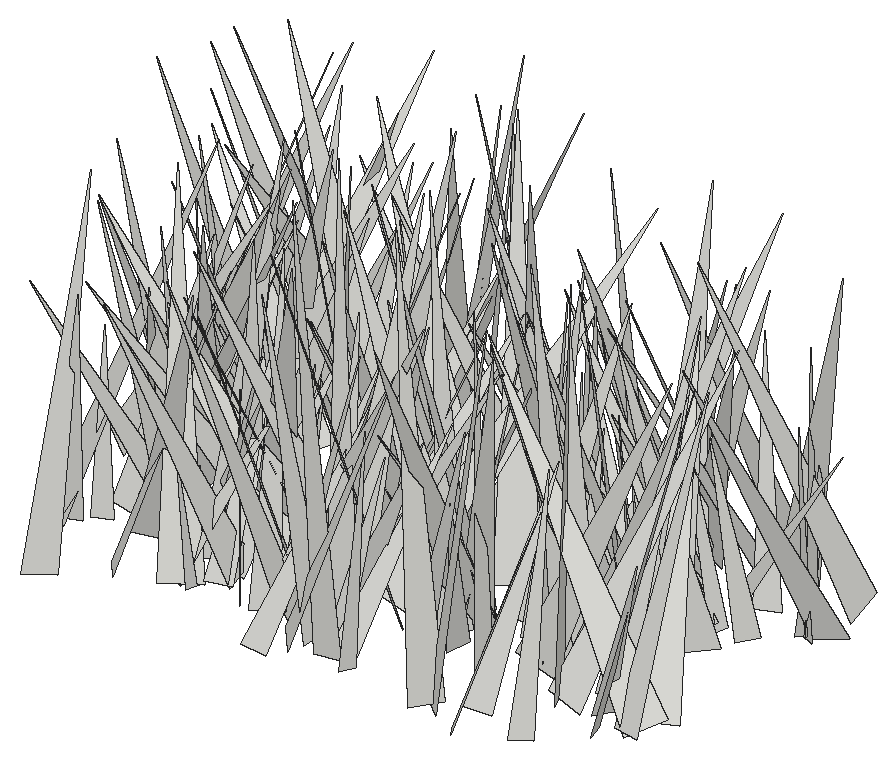
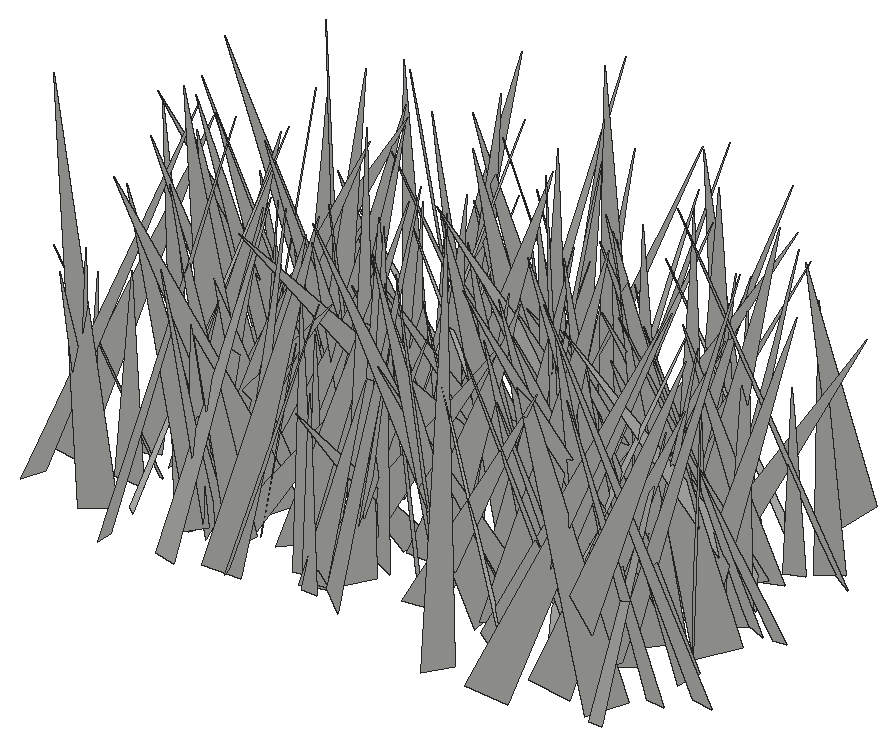
# SketchUp Ruby script. Lengths in inches.
U = 1.inch
M = Sketchup.active_model
def pt(a) = Geom::Point3d.new(a.map { |v| v * U })
def face(e, loops, mat)
  f = e.add_face(loops[0].map { |a| pt(a) })
  loops[1..].each { |l| e.add_face(l.map { |a| pt(a) }).erase! }
  f.material = f.back_material = mat if mat
  f
end
# faces: each face lists its corners as indices into pts; further lists are holes
def faces(e, pts, list, mat = nil) = list.each { |f| face(e, (f[0].is_a?(Array) ? f : [f]).map { |l| l.map { |i| pts[i] } }, mat) }
# xy, xz, yz: faces in a plane at the given z, y or x. An outline is a flat list of corners, or four numbers for a rectangle; further outlines are holes
def ring(l) = l.size == 4 ? [[l[0], l[1]], [l[2], l[1]], [l[2], l[3]], [l[0], l[3]]] : l.each_slice(2).to_a
def flat(e, list, mat, &to3) = list.each { |f| face(e, (f[0].is_a?(Array) ? f : [f]).map { |l| ring(l).map { |u, v| to3.(u, v) } }, mat) }
def xy(e, z, list, mat = nil) = flat(e, list, mat) { |x, y| [x, y, z] }
def xz(e, y, list, mat = nil) = flat(e, list, mat) { |x, z| [x, y, z] }
def yz(e, x, list, mat = nil) = flat(e, list, mat) { |y, z| [x, y, z] }
def lines(e, pts, list) = list.each { |a, b| e.add_line(pt(pts[a]), pt(pts[b])) }
# prism: a flat outline (further loops are holes) pulled along v
def prism(e, loops, v, mat = nil)
  f = face(e, loops, mat); d = Geom::Vector3d.new(v.map { |x| x * U })
  f.pushpull(f.normal.samedirection?(d) ? d.length : -d.length)
end
def box(e, o, s, mat = nil) = prism(e, [[o, [o[0] + s[0], o[1], o[2]], [o[0] + s[0], o[1] + s[1], o[2]], [o[0], o[1] + s[1], o[2]]]], [0, 0, s[2]], mat)
def at(x, y, z, deg = 0) = Geom::Transformation.translation(pt([x, y, z])) * Geom::Transformation.rotation(ORIGIN, Z_AXIS, deg.degrees)
def axes(o, x, y, z) = Geom::Transformation.new([*x, 0, *y, 0, *z, 0, *pt(o).to_a, 1])
def part(name) = M.definitions.add(name)
# library, detail: a bought-in or finely detailed component or shape, given as its bounding box
def library(name, o, s) = part(name).tap { |d| box(d.entities, o, s) }
def detail(e, o, s) = box(e.add_group.entities, o, s)
def put(e, d, t, mat = nil) = e.add_instance(d, t).tap { |i| i.material = mat if mat }
def group(e, t, mat = nil) = e.add_group.tap { |g| g.transformation = t; g.material = mat if mat }.entities
root = M.entities
c1 = part("fur_instance\#9")
p = [[0.8125,0,1.79],[0.67,-0.02,1.48],[0,-0.11,0],[0,0.11,0]]
faces(c1.entities,p,[[0,1,2,3]])
put(root,c1,axes([484.92,128.27,-21.86],[-6.34287,-0.8603,1.40577],[-0.30586,6.10717,2.3574],[1.61949,-2.21602,5.95103]))
put(root,c1,axes([487.6,127.56,-21.86],[-6.52757,-2.25287,1.08541],[-2.07972,6.57544,1.14066],[1.38863,-0.74224,6.81054]))
put(root,c1,axes([497.37,124.18,-21.86],[3.38702,2.66566,0.2184],[2.51461,-3.29384,1.20529],[-0.91115,0.81867,4.13823]))
put(root,c1,axes([488.98,125.71,-21.86],[4.58071,3.98416,0.78034],[4.05613,-4.44078,-1.1369],[0.17387,-1.36793,5.96354]))
put(root,c1,axes([489.72,126.4375,-21.86],[-6.3571,-0.05635,1.63328],[-0.03082,6.56286,0.10646],[1.63396,-0.09544,6.35645]))
put(root,c1,axes([491.91,125.34,-21.86],[-4.04138,0.55951,1.25439],[0.25517,4.13619,-1.02282],[1.34961,0.89343,3.94964]))
put(root,c1,axes([495.84,125.06,-21.86],[4.42049,5.15695,1.86392],[5.12768,-4.73588,0.94203],[-1.94301,-0.76574,6.72662]))
put(root,c1,axes([479.57,123.94,-21.86],[-6.45449,2.84921,1.13675],[2.42101,6.35763,-2.18855],[1.88385,1.59157,6.70736]))
put(root,c1,axes([480.96,128.42,-21.86],[3.49272,-6.19271,0.17705],[-6.11252,-3.41157,1.25629],[1.00898,0.76914,6.99789]))
put(root,c1,axes([493.32,127.51,-21.66],[-0.9776,-5.25666,1.94415],[-5.10339,1.65068,1.89699],[2.31681,1.41798,4.99896]))
put(root,c1,axes([499.82,124.92,-21.66],[-4.30895,1.90574,0.59057],[1.67064,4.21479,-1.41144],[1.09067,1.07302,4.49519]))
put(root,c1,axes([477.86,127.61,-21.86],[2.40691,-4.24835,1.2679],[-4.42272,-2.4014,0.34948],[-0.30924,1.27831,4.87028]))
put(root,c1,axes([490.85,125.56,-21.86],[1.70019,7.5386,2.42367],[7.33263,-2.43467,2.42902],[-2.9895,-1.68439,7.33628]))
put(root,c1,axes([495.76,124.82,-21.66],[-8.22184,1.12863,0.67504],[0.91948,7.98903,-2.15825],[0.94024,2.05661,8.01339]))
put(root,c1,axes([488.55,124.4,-21.86],[-3.43381,3.18637,0.41007],[2.54254,3.06224,-2.50406],[1.96382,1.60682,3.959]))
put(root,c1,axes([490.92,129.31,-21.86],[-4.98525,-6.36904,1.05647],[-6.36247,5.07321,0.56124],[1.09531,0.48105,8.06861]))
put(root,c1,axes([486.88,128.99,-21.86],[-4.07639,-4.57708,0.71562],[-4.52519,4.13816,0.69067],[0.99219,0.06853,6.09012]))
put(root,c1,axes([488.27,126.66,-21.86],[3.37327,4.28522,1.21914],[4.44713,-3.33099,-0.5966],[-0.2692,-1.33033,5.4209]))
put(root,c1,axes([497.16,125.85,-21.86],[-1.9043,4.31856,1.08738],[4.14528,2.15112,-1.28374],[1.62757,-0.42591,4.54184]))
put(root,c1,axes([490.35,126.78,-21.86],[-2.24113,2.46388,1.48853],[2.36542,2.65133,-0.82724],[1.6405,-0.45695,3.22631]))
put(root,c1,axes([493.4375,130.5,-21.86],[2.31085,-7.14722,0.11909],[-7.10013,-2.30949,-0.83147],[-0.82765,-0.14321,7.46535]))
put(root,c1,axes([481.29,125.78,-21.86],[4.55508,3.875,0.43107],[3.83788,-4.57312,0.55448],[-0.68713,0.14532,5.95457]))
put(root,c1,axes([486.14,126.66,-21.86],[2.37526,2.53476,1.46683],[2.25858,-2.78775,1.16004],[-1.86424,-0.14786,3.27432]))
put(root,c1,axes([483.28,126.67,-21.86],[1.22352,3.80068,0.33063],[3.61313,-1.04295,-1.38167],[1.22465,-0.72012,3.74608]))
put(root,c1,axes([493.92,128.9,-21.86],[3.65469,-1.69105,0.3912],[-1.57801,-3.61693,-0.89287],[-0.72291,-0.65395,3.92673]))
put(root,c1,axes([489.53,128.27,-21.86],[1.64693,-4.65446,0.85777],[-4.4282,-1.19483,2.01879],[1.67056,1.42146,4.50564]))
put(root,c1,axes([483.75,126.46,-21.86],[-3.76745,6.43232,1.47995],[6.58457,3.78058,0.33053],[0.45645,-1.44608,7.44709]))
put(root,c1,axes([500.65,128.38,-21.86],[3.31097,-1.72543,0.32906],[-1.73993,-3.31791,0.10944],[-0.24091,0.24944,3.73197]))
put(root,c1,axes([484.54,130.61,-21.86],[2.66865,-7.95792,0.14871],[-7.80747,-2.5868,1.68053],[1.54726,0.67254,8.22351]))
put(root,c1,axes([484.24,126.65,-21.86],[-6.19983,-0.76734,1.02255],[-1.02443,6.01091,-1.70052],[0.76483,1.83095,6.01123]))
put(root,c1,axes([491.01,126.33,-21.86],[-0.26739,4.57604,0.32256],[4.40279,0.34673,-1.26925],[1.2883,-0.2352,4.40462]))
put(root,c1,axes([488.82,130.11,-21.86],[-7.42366,-0.80204,0.92134],[-0.52005,7.2098,2.08597],[1.1053,-1.9946,7.16957]))
put(root,c1,axes([481.3125,129.65,-21.66],[0.83306,-5.07313,1.39633],[-4.3947,-1.44829,-2.63999],[-2.89363,0.73905,4.41148]))
put(root,c1,axes([483.41,128.46,-21.86],[3.19088,3.17646,1.19509],[3.39239,-3.03309,-0.99593],[-0.09903,-1.55252,4.39087]))
put(root,c1,axes([478.79,128.36,-21.86],[-1.48065,3.15767,1.46809],[3.42197,1.61497,-0.02236],[0.64523,-1.31889,3.48751]))
put(root,c1,axes([486.67,130.52,-21.86],[-3.64802,-5.0358,0.07825],[-5.03596,3.64854,0.02575],[0.06676,0.04827,6.21825]))
put(root,c1,axes([486.77,129.3125,-21.66],[2.93254,-6.52755,1.0505],[-6.19008,-2.30697,2.94501],[2.32281,2.09313,6.52193]))
put(root,c1,axes([493.27,130.65,-21.86],[0.69431,-7.1025,1.01226],[-6.95299,-0.41552,1.85354],[1.7681,1.15502,6.89145]))
put(root,c1,axes([502.45,128.47,-21.86],[-5.51381,4.9525,0.02994],[4.6746,5.18943,2.47955],[-1.63592,-1.86355,6.98435]))
put(root,c1,axes([483.41,131.8,-21.86],[-6.30471,-1.37126,0.42808],[-1.05468,5.72683,2.8114],[0.97532,-2.67133,5.80738]))
put(root,c1,axes([480.91,129.66,-21.86],[-6.26748,-0.84521,1.62615],[-0.68504,6.45447,0.7145],[1.69984,-0.51518,6.28372]))
put(root,c1,axes([501.47,126.89,-21.66],[5.51365,3.20537,1.24598],[2.89904,-5.59864,1.57419],[-1.84998,0.77981,6.18035]))
put(root,c1,axes([486.14,130.14,-21.66],[-7.10232,2.48969,0.17848],[2.39972,6.66255,2.55443],[-0.68683,-2.46683,7.07929]))
put(root,c1,axes([482.45,129.63,-21.66],[1.69765,-3.69471,0.41656],[-3.54176,-1.46758,1.41724],[1.13153,0.9496,3.81108]))
put(root,c1,axes([498.7,128.42,-21.86],[6.19858,3.66698,3.16063],[3.75526,-6.8827,0.6206],[-3.05522,-1.01998,7.17523]))
put(root,c1,axes([487.97,127.2,-21.86],[-3.80527,0.70423,0.62745],[0.3357,3.44844,-1.83447],[0.88144,1.72686,3.40746]))
put(root,c1,axes([489.45,128.6,-21.86],[3.70489,5.29932,0.63458],[5.07029,-3.25343,-2.43293],[1.66665,-1.88258,5.99082]))
put(root,c1,axes([487.15,126.79,-21.86],[-5.93651,2.05948,0.4431],[1.83167,5.70073,-1.95618],[1.04056,1.71471,5.97135]))
put(root,c1,axes([488.66,128.81,-21.86],[-2.20726,4.7722,2.01563],[5.04733,2.47451,-0.33147],[1.16667,-1.67676,5.24748]))
put(root,c1,axes([492.56,132.53,-21.86],[-3.99829,-3.957,0.07334],[-3.50173,3.58563,2.55553],[1.84422,-1.77059,5.01133]))
put(root,c1,axes([490.3,127.07,-21.66],[1.13757,8.04859,1.54719],[7.76789,-1.55698,2.3882],[-2.61411,-1.12413,7.76984]))
put(root,c1,axes([482.25,129.13,-21.86],[-1.59145,-6.67923,2.98055],[-7.18236,0.85085,-1.92829],[-1.38185,3.26993,6.58988]))
put(root,c1,axes([477.29,127.72,-21.86],[4.54632,6.46757,0.61256],[6.48609,-4.47646,-0.87508],[0.36794,-1.0028,7.85702]))
put(root,c1,axes([487.18,127.6,-21.66],[-2.89965,3.32427,1.06428],[2.78447,3.03733,-1.90073],[2.1048,0.5615,3.98069]))
put(root,c1,axes([496.72,129.56,-21.86],[2.05152,-6.6713,2.37008],[-6.64568,-0.96384,3.03943],[2.44098,2.98279,6.28306]))
put(root,c1,axes([487.1,128.23,-21.86],[-3.85021,0.78609,0.9669],[0.45373,3.80886,-1.28983],[1.16059,1.11875,3.71193]))
put(root,c1,axes([496,127.7,-21.66],[-6.18556,-0.57175,1.0735],[-0.94708,5.75521,-2.39186],[0.76312,2.5082,5.73298]))
put(root,c1,axes([484.51,128.31,-21.86],[0.05703,4.78722,0.58826],[4.57544,0.13244,-1.52137],[1.52606,-0.57598,4.5394]))
put(root,c1,axes([483.98,129.87,-21.86],[5.0258,-2.8928,2.35137],[-3.11716,-5.42578,-0.01254],[-2.04464,1.16127,5.79886]))
put(root,c1,axes([484.75,127.26,-21.86],[-4.05374,2.9207,0.15477],[2.65047,3.78022,-1.91631],[1.23673,1.47198,4.61422]))
put(root,c1,axes([500.62,130.41,-21.86],[-4.58076,1.47717,0.18742],[1.47131,4.39705,1.30451],[-0.22897,-1.29786,4.63288]))
put(root,c1,axes([502.125,127.76,-21.86],[1.80185,5.93958,0.37976],[5.89361,-1.83593,0.75111],[-0.82954,-0.14229,6.16126]))
put(root,c1,axes([481.49,132.89,-21.86],[5.03177,-2.92165,1.14225],[-2.20313,-4.82824,-2.64459],[-2.23316,-1.81978,5.18275]))
put(root,c1,axes([478.05,132.35,-21.86],[5.48383,-1.63022,0.30334],[-1.45467,-5.23263,-1.82362],[-0.79597,-1.66854,5.42259]))
put(root,c1,axes([494.63,130.01,-21.66],[-7.44301,-3.63877,0.95843],[-3.76282,7.20814,-1.85509],[0.01898,2.08796,8.0745]))
put(root,c1,axes([480.19,132.4375,-21.86],[6.15158,-3.29467,0.71793],[-3.15743,-6.15236,-1.17953],[-1.18361,-0.7112,6.87789]))
put(root,c1,axes([479.05,129.32,-21.86],[0.12132,5.40428,1.16344],[5.42728,0.10479,-1.05269],[1.05091,-1.16504,5.30215]))
put(root,c1,axes([498.42,132.28,-21.66],[2.63611,-2.6678,0.56163],[-2.26437,-2.5776,-1.61563],[-1.51829,-0.78771,3.38467]))
put(root,c1,axes([497.59,130.51,-21.86],[-7.11208,1.53537,2.26223],[1.65379,7.4363,0.15223],[2.17716,-0.6331,7.27433]))
put(root,c1,axes([497.73,130.75,-21.86],[3.10657,-5.20372,2.6425],[-5.63717,-3.45056,-0.16782],[-1.51121,2.17421,6.05816]))
put(root,c1,axes([489.14,128.73,-21.66],[-5.55671,4.70477,2.20019],[4.40361,5.97611,-1.65743],[2.7539,-0.06297,7.08977]))
put(root,c1,axes([499.12,128.16,-21.86],[1.06363,7.1406,0.14161],[6.98782,-1.01087,-1.51263],[1.47601,-0.35985,7.05914]))
put(root,c1,axes([497.95,130.64,-21.86],[5.04993,-3.13211,0.88061],[-3.25342,-4.87587,1.31476],[-0.02926,1.58216,5.79512]))
put(root,c1,axes([487.84,126.92,-21.86],[6.81061,4.1437,0.72104],[3.52808,-6.3754,3.31382],[-2.28972,2.50169,7.25074]))
put(root,c1,axes([483.64,128.67,-21.86],[-6.63675,3.07759,1.929],[2.57186,6.8191,-2.03087],[2.56478,1.12578,7.02806]))
put(root,c1,axes([500.14,130.71,-21.86],[-5.99226,-3.56649,1.99916],[-3.93709,5.99,-1.11487],[1.10264,2.00593,6.88361]))
put(root,c1,axes([491.8,131.28,-21.86],[-4.16416,5.80884,2.0419],[6.1268,3.66414,2.07088],[-0.6118,-2.84317,6.84063]))
put(root,c1,axes([495.84,133.73,-21.86],[-0.44109,-6.89492,0.21564],[-6.89758,0.44393,0.08524],[0.09888,0.20974,6.90849]))
put(root,c1,axes([479.54,130.57,-21.86],[6.84085,-1.05323,0.60817],[-1.14548,-6.7472,1.19982],[-0.40871,1.28156,6.81667]))
put(root,c1,axes([500.33,129.26,-21.86],[1.00933,7.00307,0.82634],[7.04916,-1.02422,0.06983],[-0.18746,-0.80782,7.07509]))
put(root,c1,axes([479.53,129.73,-21.86],[-0.99691,5.86129,1.26655],[5.41282,1.43213,-2.36709],[2.58075,-0.73958,5.45394]))
put(root,c1,axes([497.22,131.01,-21.86],[2.53545,-3.02814,1.98338],[-3.53036,-2.60371,0.53779],[-0.80002,1.89288,3.91266]))
put(root,c1,axes([500.49,131.82,-21.86],[-2.5015,-6.23633,1.72664],[-6.18785,1.76379,-2.59425],[-1.89304,2.47545,6.19832]))
put(root,c1,axes([502.52,129.04,-21.86],[-3.69849,5.78351,0.10997],[5.76561,3.69627,-0.48502],[0.46777,0.16892,6.84781]))
put(root,c1,axes([479.17,133.25,-21.86],[-0.56263,-5.96411,0.83016],[-5.9756,0.45013,-0.816],[-0.74291,0.89616,5.93475]))
put(root,c1,axes([493.37,129.42,-21.66],[-7.58228,1.17889,0.51367],[1.00041,7.33787,-2.07353],[0.80796,1.97752,7.38791]))
put(root,c1,axes([487.95,131.51,-21.86],[5.05169,2.87341,0.23488],[2.86098,-4.93803,-1.1233],[0.35552,-1.09113,5.70213]))
put(root,c1,axes([493.51,129.47,-21.66],[3.73526,4.02595,0.93613],[3.5763,-3.78049,1.98866],[-2.07237,0.73241,5.11915]))
put(root,c1,axes([487.65,134.23,-21.86],[-4.40501,-3.46188,0.56585],[-3.18391,4.32713,1.68747],[1.47225,-1.00011,5.34239]))
put(root,c1,axes([496.63,129.85,-21.86],[3.23969,5.31398,1.47982],[4.81259,-3.56155,2.25346],[-2.69577,0.02794,5.80137]))
put(root,c1,axes([487.27,132.4,-21.86],[-5.96506,-5.04673,2.13711],[-5.35643,6.03696,-0.69462],[1.15994,1.92465,7.7826]))
put(root,c1,axes([479.91,131.73,-21.86],[1.06055,3.50039,1.15885],[3.68372,-1.05849,-0.17402],[-0.16095,-1.16074,3.65339]))
put(root,c1,axes([498.75,132.47,-21.86],[-3.07228,-3.20464,1.70758],[-3.41257,3.31254,0.07678],[1.24093,1.17551,4.43878]))
put(root,c1,axes([486.8,133.02,-21.86],[4.6953,-3.04636,0.27903],[-3.0591,-4.67738,0.40996],[-0.01004,0.49581,5.58194]))
put(root,c1,axes([489.04,129.92,-21.66],[-0.72981,5.66267,0.18679],[5.27184,0.7477,-2.06932],[2.0757,0.09199,5.32132]))
put(root,c1,axes([494.92,131.33,-21.66],[0.03903,6.40601,1.64221],[6.43648,0.34027,-1.48032],[1.51842,-1.60705,6.23275]))
put(root,c1,axes([491.09,131.02,-21.66],[4.64309,0.99306,0.50279],[0.80416,-4.48393,1.43003],[-0.7696,1.30595,4.52764]))
put(root,c1,axes([495.22,132.98,-21.86],[-1.62958,-3.15436,1.09529],[-3.33909,1.53504,-0.54711],[-0.01197,1.22427,3.50802]))
put(root,c1,axes([484.9,133.61,-21.86],[6.58164,2.52237,2.667],[2.99732,-6.85363,-0.91486],[-2.11926,-1.85972,6.9888]))
put(root,c1,axes([500.53,133.87,-21.86],[-3.08305,4.83073,2.80211],[5.58378,2.72141,1.452],[0.09585,-3.15451,5.54372]))
put(root,c1,axes([499.12,132.52,-21.86],[-4.22119,3.06488,0.48562],[3.10212,4.18863,0.52921],[0.07866,-0.71394,5.1896]))
put(root,c1,axes([483.28,133.63,-21.66],[-3.66042,-4.84933,0.70173],[-4.78346,3.34689,-1.82316],[-1.06154,1.63996,5.79575]))
put(root,c1,axes([477.4,134.24,-21.86],[4.73655,-6.32836,0.37656],[-6.13582,-4.45802,2.25891],[1.59428,1.644,7.57499]))
put(root,c1,axes([479.45,134.45,-21.86],[0.83878,-6.84447,1.51714],[-6.71971,-0.34936,2.13903],[1.99848,1.69801,6.55552]))
put(root,c1,axes([482.21,132.85,-21.66],[1.25839,-5.65908,2.69216],[-6.0262,-0.33916,2.10388],[1.71982,2.95233,5.40207]))
put(root,c1,axes([476.01,132.61,-21.66],[3.46284,5.45761,0.55951],[5.19477,-3.049,-2.40992],[1.76435,-1.73432,5.99742]))
put(root,c1,axes([477.37,132.25,-21.86],[3.14685,5.37097,0.90824],[5.43729,-3.03382,-0.89816],[0.32882,-1.23429,6.15981]))
put(root,c1,axes([480.875,134.83,-21.86],[2.63547,-2.52355,0.88422],[-2.24578,-2.7628,-1.19134],[-1.45143,-0.30736,3.44888]))
put(root,c1,axes([486.22,135.1,-21.66],[-4.22859,-0.79072,0.99748],[-0.41595,4.12901,1.5098],[1.20299,-1.35177,4.02824]))
put(root,c1,axes([486.1,135.52,-21.86],[0.0355,-6.28923,0.69696],[-6.32457,-0.05728,-0.19472],[-0.19984,0.69551,6.28631]))
put(root,c1,axes([481.9,132.51,-21.86],[-6.30755,-1.0303,0.95825],[-1.23667,6.15876,-1.51833],[0.67114,1.66527,6.20817]))
put(root,c1,axes([495.81,130.73,-21.66],[-6.32088,1.55628,0.92222],[1.03646,5.86264,-2.78949],[1.48264,2.53644,5.88169]))
put(root,c1,axes([483.86,132.52,-21.86],[-4.16837,-0.36819,0.02902],[-0.35612,3.91965,-1.4217],[-0.09791,1.41863,3.93569]))
put(root,c1,axes([496.86,133.83,-21.66],[-1.92463,-5.23066,1.71698],[-5.26178,1.21283,-2.20335],[-1.6191,2.27625,5.1195]))
put(root,c1,axes([493.3,135.97,-21.86],[-1.0754,-7.3325,1.08617],[-7.40599,1.10888,0.15329],[0.31086,1.05196,7.40935]))
put(root,c1,axes([487.26,136.06,-21.86],[3.85472,-3.45884,0.89823],[-3.26491,-3.94586,-1.18314],[-1.45282,-0.30973,5.04209]))
put(root,c1,axes([490.16,129.9,-21.86],[-4.06981,7.2471,0.38585],[5.9474,3.58401,-4.58433],[4.15906,1.9665,6.9331]))
put(root,c1,axes([503.5,137.29,-21.86],[1.05272,-6.58483,0.46236],[-6.33643,-1.13928,-1.79827],[-1.85027,0.15508,6.42141]))
put(root,c1,axes([478.94,130.22,-21.66],[6.66219,5.05954,0.23915],[4.47229,-6.06129,3.64695],[-2.37798,2.77537,7.52884]))
put(root,c1,axes([478.16,134.75,-21.86],[3.3067,2.95122,2.18217],[3.23124,-3.73382,0.15332],[-1.74087,-1.32466,4.4295]))
put(root,c1,axes([501.29,135.47,-21.86],[2.35364,-2.97334,1.61897],[-3.0072,-2.74184,-0.66374],[-1.55518,0.80187,3.73361]))
put(root,c1,axes([497.86,136.96,-21.86],[1.37303,-5.10418,0.31363],[-5.09334,-1.39399,-0.38851],[-0.45708,0.20095,5.27134]))
put(root,c1,axes([486.45,133.57,-21.66],[6.53232,-2.04401,3.08815],[-2.89411,-6.72439,1.67109],[-2.31057,2.64395,6.63752]))
put(root,c1,axes([494.82,134.42,-21.86],[1.15906,3.62365,1.13013],[3.60388,-1.42153,0.86183],[-1.19166,-0.77453,3.7056]))
put(root,c1,axes([496.82,133.9,-21.66],[0.16958,6.97336,1.46095],[6.91324,0.19239,-1.72074],[1.72314,-1.45812,6.75984]))
put(root,c1,axes([479.39,137.17,-21.66],[-7.48109,-1.28394,1.71532],[-0.94889,7.57103,1.5286],[1.92105,-1.26035,7.43496]))
put(root,c1,axes([499.0625,139.22,-21.66],[-5.37416,-4.85351,0.14678],[-4.51514,5.07548,2.5125],[1.7865,-1.77274,6.79157]))
put(root,c1,axes([498.51,134.4,-21.86],[5.95771,-4.00613,4.25574],[-5.13988,-6.48421,1.09155],[-2.78246,3.40011,7.09591]))
put(root,c1,axes([479.39,137.04,-21.86],[2.07111,-6.85146,1.31632],[-6.80663,-1.68294,1.94991],[1.53132,1.78604,6.88693]))
put(root,c1,axes([500.14,135.32,-21.86],[-4.0966,0.35691,0.30901],[0.31396,4.07547,-0.54495],[0.35257,0.51784,4.07585]))
put(root,c1,axes([495.61,137.42,-21.86],[-0.91918,-4.72146,0.08029],[-4.18667,0.777,-2.23865],[-2.18412,0.49761,4.25741]))
put(root,c1,axes([488.07,135.07,-21.86],[-5.27526,-0.92635,0.94955],[-1.13263,5.17215,-1.24665],[0.69057,1.40673,5.20887]))
put(root,c1,axes([496.81,138.21,-21.86],[2.5877,-3.76016,0.15432],[-3.53923,-2.49522,-1.45139],[-1.27925,-0.70276,4.32764]))
put(root,c1,axes([492.74,133.54,-21.86],[-7.32021,3.8589,0.48336],[3.73123,7.2592,-1.44642],[1.09666,1.05977,8.14767]))
put(root,c1,axes([499.61,135.07,-21.86],[-2.18408,5.95276,0.46734],[5.01759,1.55993,3.57972],[-3.2369,-1.59851,5.23366]))
put(root,c1,axes([482.9375,136.49,-21.66],[-5.86461,-3.9483,0.52207],[-3.9663,5.70596,-1.40208],[-0.36068,1.452,6.92942]))
put(root,c1,axes([496.57,139.03,-21.66],[-0.05965,-7.49908,0.31223],[-6.76708,0.1888,3.24163],[3.24657,0.25574,6.76251]))
put(root,c1,axes([479.4,135.16,-21.86],[0.42432,7.03314,2.02201],[6.63788,0.48281,-3.07232],[3.08094,-2.00885,6.34082]))
put(root,c1,axes([477.05,136.31,-21.86],[4.99939,-0.31235,0.02616],[-0.31267,-4.999,0.06629],[-0.02197,0.06779,5.0087]))
put(root,c1,axes([493.22,137.7,-21.66],[-6.6748,0.96554,1.83268],[1.43583,6.61336,1.7452],[1.49311,-2.0433,6.51456]))
put(root,c1,axes([489.83,138.3,-21.66],[7.80174,-0.94154,1.76979],[-0.49694,-7.7978,-1.95786],[-1.94209,-1.78708,7.61055]))
put(root,c1,axes([481.73,136.32,-21.66],[-4.33384,4.15795,0.46311],[4.09626,4.08164,1.68703],[-0.85069,-1.52868,5.76409]))
put(root,c1,axes([484.22,135.02,-21.86],[0.04484,6.03011,0.93276],[6.10111,-0.02998,-0.09948],[0.09373,-0.93336,6.02946]))
put(root,c1,axes([499.67,136.83,-21.66],[3.27011,3.05252,0.13659],[2.8317,-2.95233,-1.81533],[1.14804,-1.41282,4.08853]))
put(root,c1,axes([491.82,136.77,-21.86],[-2.20634,6.02099,1.75888],[5.48729,0.94934,3.63349],[-3.03901,-2.65713,5.28374]))
put(root,c1,axes([488.88,135.6875,-21.66],[-3.57557,6.64036,0.56629],[6.42877,3.26724,2.27945],[-1.75672,-1.55901,7.1891]))
put(root,c1,axes([490.76,139.01,-21.86],[3.46257,-3.0651,1.27719],[-2.41097,-3.5895,-2.07802],[-2.28326,-0.85797,4.13111]))
put(root,c1,axes([481.46,135.55,-21.86],[-0.62472,6.74476,1.37593],[6.88336,0.62526,0.06028],[0.06565,-1.37569,6.77336]))
put(root,c1,axes([485.56,134.97,-21.86],[-0.37436,5.47936,0.25355],[5.20879,0.43477,-1.70506],[1.71934,-0.12411,5.22075]))
put(root,c1,axes([502.86,136.76,-21.86],[1.66971,3.21733,1.57549],[3.35444,-2.01427,0.55833],[-1.25742,-1.10127,3.58153]))
put(root,c1,axes([503.21,139.41,-21.66],[-7.55604,-1.18176,1.01335],[-0.88861,7.39753,2.00103],[1.27821,-1.84315,7.38147]))
put(root,c1,axes([479.98,134.19,-21.66],[0.04279,8.23701,0.26485],[7.98617,0.02394,-2.03491],[2.0346,-0.26721,7.98181]))
put(root,c1,axes([484.01,137.57,-21.66],[-5.61004,5.72169,2.32507],[6.16954,5.3361,1.75473],[0.28367,-2.89906,7.81865]))
put(root,c1,axes([490.49,136.54,-21.86],[1.87849,6.8023,2.53671],[7.02619,-2.36292,1.13321],[-1.82724,-2.09291,6.96533]))
put(root,c1,axes([495.03,137.13,-21.86],[-3.64875,-2.02244,1.121],[-2.25149,3.58457,-0.86132],[0.52696,1.3118,4.08188]))
put(root,c1,axes([496.12,136.54,-21.66],[-7.03444,-1.19576,1.59787],[-1.52444,6.99776,-1.47438],[1.28808,1.75153,6.98136]))
put(root,c1,axes([481.76,141.45,-21.86],[4.2838,-6.03866,0.74714],[-5.20831,-4.11147,-3.36808],[-3.14598,-1.41597,6.59337]))
put(root,c1,axes([490.02,134.96,-21.66],[-3.33289,3.23483,0.32122],[2.5841,2.91556,-2.549],[1.97223,1.64647,3.88264]))
put(root,c1,axes([491,136.99,-21.86],[-4.99068,-1.45127,1.21381],[-1.71677,4.91279,-1.18474],[0.79513,1.49823,5.06058]))
put(root,c1,axes([491.86,138.77,-21.86],[-0.19463,-4.95849,1.24268],[-5.00803,0.4343,0.94858],[1.02496,1.18047,4.8708]))
put(root,c1,axes([488.43,136.82,-21.86],[4.10758,4.73433,2.04961],[4.7509,-4.49256,0.85604],[-2.01089,-0.9434,6.20913]))
put(root,c1,axes([494.875,138.37,-21.86],[6.50661,-0.43072,0.76621],[-0.39332,-6.54513,-0.33931],[-0.78607,-0.29036,6.51202]))
put(root,c1,axes([479.74,137.96,-21.66],[2.31497,4.33574,1.17317],[4.28428,-1.73503,-2.04175],[1.34907,-1.93005,4.47091]))
put(root,c1,axes([496.3,140.85,-21.86],[-2.87377,-5.9267,0.11201],[-5.79461,2.83495,1.33509],[1.24935,-0.48389,6.44995]))
put(root,c1,axes([495.3,135.86,-21.86],[-3.36255,6.42423,2.20976],[5.77924,4.00105,-2.8377],[3.57129,-0.42595,6.67271]))
put(root,c1,axes([498.38,136.29,-21.66],[-4.64664,1.60589,0.29185],[1.45378,4.47236,-1.46283],[0.74202,1.29401,4.69365]))
put(root,c1,axes([496.52,138.16,-21.86],[4.99795,-3.82327,1.26682],[-4.01963,-4.86241,1.18375],[-0.25457,1.71502,6.18026]))
put(root,c1,axes([502.72,137.2,-21.86],[-4.80095,-0.85986,1.55653],[-1.24807,4.82151,-1.18603],[1.26668,1.49164,4.73094]))
put(root,c1,axes([494.21,140.39,-21.86],[1.78326,-6.33726,0.7797],[-6.26284,-1.89367,-1.06754],[-1.24322,0.44943,6.49625]))
put(root,c1,axes([477.62,140.6875,-21.86],[-2.3415,-4.6423,0.1365],[-4.37976,2.25803,1.66471],[1.54509,-0.63449,4.92568]))
put(root,c1,axes([498.58,141.3125,-21.66],[-6.83559,-3.49227,1.59422],[-2.83471,6.78714,2.71329],[2.5888,-1.7893,7.18049]))
put(root,c1,axes([500.5625,137.46,-21.86],[-0.93822,4.8343,1.08723],[4.93478,0.81164,0.64956],[-0.44769,-1.18472,4.88147]))
put(root,c1,axes([483.3,139.17,-21.66],[-3.35024,-7.10363,1.41562],[-6.97339,2.74138,-2.74705],[-1.95891,2.39017,7.35795]))
put(root,c1,axes([500.04,139.85,-21.66],[1.15039,-7.47242,1.55869],[-7.41634,-0.72104,2.01691],[1.80677,1.79806,7.28646]))
put(root,c1,axes([475.38,137.63,-21.66],[3.97232,6.71602,1.21655],[6.692,-3.55551,-2.22255],[1.34242,-2.14887,7.47961]))
put(root,c1,axes([489.97,139.625,-21.86],[4.25123,5.18566,4.75994],[6.35301,-5.22113,0.01405],[-3.03108,-3.67013,6.70551]))
put(root,c1,axes([485.14,136.98,-21.86],[8.11647,0.24258,0.67526],[0.10402,-7.98511,1.61836],[-0.70993,1.60345,7.95719]))
put(root,c1,axes([487.2,138.28,-21.66],[-4.10469,4.34568,0.4298],[4.19686,3.76273,2.03626],[-1.20665,-1.6956,5.62024]))
put(root,c1,axes([480.36,137.97,-21.66],[3.62784,4.7769,0.79864],[4.78599,-3.38301,-1.50576],[0.74217,-1.53438,5.80626]))
put(root,c1,axes([482.87,139.08,-21.66],[5.29628,3.42643,1.15131],[3.61426,-4.98862,-1.7797],[0.0553,-2.11891,6.05175]))
put(root,c1,axes([476.89,138.33,-21.86],[2.54446,5.11145,1.43196],[5.2695,-2.24073,-1.36501],[0.64019,-1.87187,5.54418]))
put(root,c1,axes([502.59,136.88,-21.86],[-4.99347,0.21503,1.45697],[-0.36457,4.80955,-1.95935],[1.42691,1.98134,4.59803]))
put(root,c1,axes([491.11,139.28,-21.86],[-2.91756,2.69263,1.56889],[3.08399,2.80363,0.92331],[0.448,-1.76443,3.86133]))
put(root,c1,axes([480.32,139.84,-21.86],[1.0703,-6.74535,2.51722],[-6.58595,-1.94546,-2.41292],[-2.90886,1.9228,6.3893]))
put(root,c1,axes([494.09,140.08,-21.86],[-4.72142,-2.258,0.83052],[-2.14472,4.77905,0.80066],[1.09019,-0.37724,5.17198]))
put(root,c1,axes([487.13,136.51,-21.66],[-7.34355,0.30763,3.29021],[-0.75169,7.65215,-2.39318],[3.21793,2.48952,6.94946]))
put(root,c1,axes([486.54,137.94,-21.86],[4.33311,5.30156,2.10924],[5.44411,-4.63436,0.46433],[-1.70794,-1.32191,6.83131]))
put(root,c1,axes([477.92,139.67,-21.86],[6.5822,-3.48627,0.04021],[-3.46978,-6.5418,0.80411],[0.34104,0.72931,7.40492]))
put(root,c1,axes([484.18,141.08,-21.86],[7.49694,-1.26912,1.50095],[-0.87324,-7.45265,-1.93987],[-1.76095,-1.70734,7.35199]))
put(root,c1,axes([496.27,138.35,-21.86],[4.8135,2.02359,1.54657],[1.94555,-5.05552,0.55956],[-1.64367,-0.05793,5.19149]))
put(root,c1,axes([490.94,139.64,-21.86],[-0.48959,-3.44443,1.08487],[-3.54488,0.6673,0.51889],[0.68909,0.98557,3.44014]))
